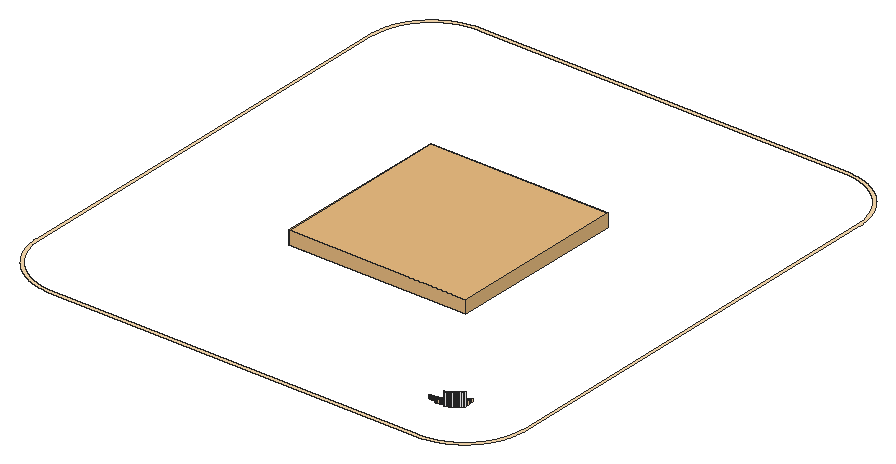
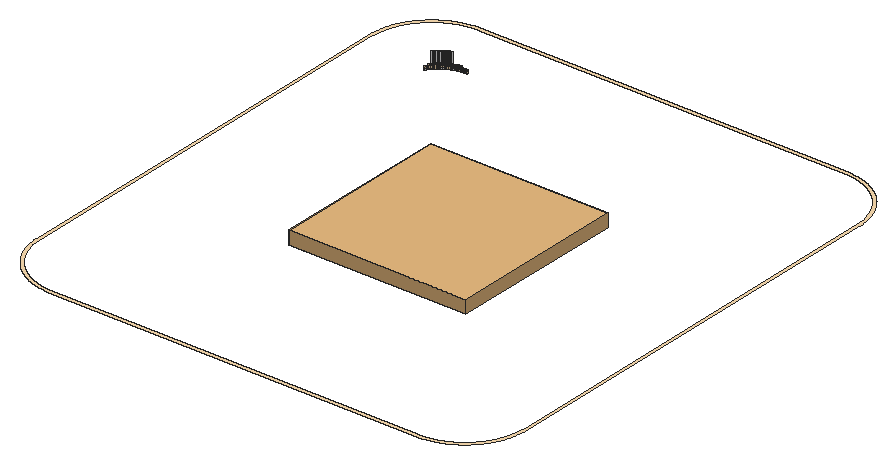
# SketchUp Ruby script. Lengths in inches.
U = 1.inch
M = Sketchup.active_model
def pt(a) = Geom::Point3d.new(a.map { |v| v * U })
def face(e, loops, mat)
  f = e.add_face(loops[0].map { |a| pt(a) })
  loops[1..].each { |l| e.add_face(l.map { |a| pt(a) }).erase! }
  f.material = f.back_material = mat if mat
  f
end
# faces: each face lists its corners as indices into pts; further lists are holes
def faces(e, pts, list, mat = nil) = list.each { |f| face(e, (f[0].is_a?(Array) ? f : [f]).map { |l| l.map { |i| pts[i] } }, mat) }
# xy, xz, yz: faces in a plane at the given z, y or x. An outline is a flat list of corners, or four numbers for a rectangle; further outlines are holes
def ring(l) = l.size == 4 ? [[l[0], l[1]], [l[2], l[1]], [l[2], l[3]], [l[0], l[3]]] : l.each_slice(2).to_a
def flat(e, list, mat, &to3) = list.each { |f| face(e, (f[0].is_a?(Array) ? f : [f]).map { |l| ring(l).map { |u, v| to3.(u, v) } }, mat) }
def xy(e, z, list, mat = nil) = flat(e, list, mat) { |x, y| [x, y, z] }
def xz(e, y, list, mat = nil) = flat(e, list, mat) { |x, z| [x, y, z] }
def yz(e, x, list, mat = nil) = flat(e, list, mat) { |y, z| [x, y, z] }
def lines(e, pts, list) = list.each { |a, b| e.add_line(pt(pts[a]), pt(pts[b])) }
# prism: a flat outline (further loops are holes) pulled along v
def prism(e, loops, v, mat = nil)
  f = face(e, loops, mat); d = Geom::Vector3d.new(v.map { |x| x * U })
  f.pushpull(f.normal.samedirection?(d) ? d.length : -d.length)
end
def box(e, o, s, mat = nil) = prism(e, [[o, [o[0] + s[0], o[1], o[2]], [o[0] + s[0], o[1] + s[1], o[2]], [o[0], o[1] + s[1], o[2]]]], [0, 0, s[2]], mat)
def at(x, y, z, deg = 0) = Geom::Transformation.translation(pt([x, y, z])) * Geom::Transformation.rotation(ORIGIN, Z_AXIS, deg.degrees)
def axes(o, x, y, z) = Geom::Transformation.new([*x, 0, *y, 0, *z, 0, *pt(o).to_a, 1])
def part(name) = M.definitions.add(name)
# library, detail: a bought-in or finely detailed component or shape, given as its bounding box
def library(name, o, s) = part(name).tap { |d| box(d.entities, o, s) }
def detail(e, o, s) = box(e.add_group.entities, o, s)
def put(e, d, t, mat = nil) = e.add_instance(d, t).tap { |i| i.material = mat if mat }
def group(e, t, mat = nil) = e.add_group.tap { |g| g.transformation = t; g.material = mat if mat }.entities
root = M.entities
M.materials.add("False Ceiling Light").color = [254, 223, 179]
M.materials.add("[Quartz Light Grey]").color = [251, 251, 252]
c1 = library("Group\#76",[0,0,0],[64,64,5])
xy(root,116.49,[[[44.53,43.5,177.47,43.5,177.71,43.51,177.94,43.52,178.18,43.53,178.41,43.54,178.65,43.56,178.88,43.58,179.12,43.6,179.35,43.625,179.59,43.65,180.05,43.71,180.29,43.74,180.98,43.86,181.22,43.9,181.45,43.94,182.14,44.09,182.6,44.21,182.82,44.27,183.28,44.39,183.5,44.46,183.73,44.53,183.95,44.6,184.18,44.68,184.4,44.75,184.84,44.91,185.0625,44.99,185.28,45.08,185.72,45.26,185.9375,45.35,186.15,45.45,186.37,45.54,186.79,45.74,187,45.85,187.21,45.95,187.84,46.28,188.05,46.4,188.25,46.51,188.45,46.63,188.66,46.75,188.86,46.88,189.06,47,189.25,47.13,189.65,47.39,189.84,47.52,190.03,47.66,190.23,47.8,190.42,47.9375,190.6,48.08,190.79,48.22,190.98,48.37,191.16,48.51,191.52,48.81,191.7,48.97,191.88,49.12,192.06,49.28,192.23,49.4375,192.4,49.6,192.74,49.92,193.08,50.26,193.4,50.6,193.5625,50.77,193.72,50.94,193.88,51.12,194.03,51.3,194.19,51.48,194.49,51.84,194.63,52.02,194.78,52.21,194.92,52.4,195.0625,52.58,195.2,52.77,195.34,52.97,195.48,53.16,195.61,53.35,195.87,53.75,196,53.94,196.12,54.14,196.25,54.34,196.37,54.55,196.49,54.75,196.6,54.95,196.72,55.16,197.05,55.79,197.15,56,197.26,56.21,197.46,56.63,197.55,56.85,197.65,57.0625,197.74,57.28,197.92,57.72,198.01,57.9375,198.09,58.16,198.25,58.6,198.32,58.82,198.4,59.05,198.47,59.27,198.54,59.5,198.61,59.72,198.73,60.18,198.79,60.4,198.91,60.86,199.06,61.55,199.1,61.78,199.14,62.02,199.26,62.71,199.29,62.95,199.35,63.41,199.375,63.65,199.4,63.88,199.42,64.12,199.44,64.35,199.46,64.59,199.47,64.82,199.48,65.06,199.49,65.29,199.5,65.53,199.5,216.47,199.49,216.71,199.48,216.94,199.47,217.18,199.46,217.41,199.44,217.65,199.42,217.88,199.4,218.12,199.375,218.35,199.35,218.59,199.29,219.05,199.26,219.29,199.14,219.98,199.1,220.22,199.06,220.45,198.91,221.14,198.79,221.6,198.73,221.82,198.61,222.28,198.54,222.5,198.47,222.73,198.4,222.95,198.32,223.18,198.25,223.4,198.09,223.84,198.01,224.0625,197.92,224.28,197.74,224.72,197.65,224.9375,197.55,225.15,197.46,225.37,197.26,225.79,197.15,226,197.05,226.21,196.72,226.84,196.6,227.05,196.49,227.25,196.37,227.45,196.25,227.66,196.12,227.86,196,228.06,195.87,228.25,195.61,228.65,195.48,228.84,195.34,229.03,195.2,229.23,195.0625,229.42,194.92,229.6,194.78,229.79,194.63,229.98,194.49,230.16,194.19,230.52,194.03,230.7,193.88,230.88,193.72,231.06,193.5625,231.23,193.4,231.4,193.08,231.74,192.74,232.08,192.4,232.4,192.23,232.5625,192.06,232.72,191.88,232.88,191.7,233.03,191.52,233.19,191.16,233.49,190.98,233.63,190.79,233.78,190.6,233.92,190.42,234.0625,190.23,234.2,190.03,234.34,189.84,234.48,189.65,234.61,189.25,234.87,189.06,235,188.86,235.12,188.66,235.25,188.45,235.37,188.25,235.49,188.05,235.6,187.84,235.72,187.21,236.05,187,236.15,186.79,236.26,186.37,236.46,186.15,236.55,185.9375,236.65,185.72,236.74,185.28,236.92,185.0625,237.01,184.84,237.09,184.4,237.25,184.18,237.32,183.95,237.4,183.73,237.47,183.5,237.54,183.28,237.61,182.82,237.73,182.6,237.79,182.14,237.91,181.45,238.06,181.22,238.1,180.98,238.14,180.29,238.26,180.05,238.29,179.59,238.35,179.35,238.375,179.12,238.4,178.88,238.42,178.65,238.44,178.41,238.46,178.18,238.47,177.94,238.48,177.71,238.49,177.47,238.5,44.53,238.5,44.29,238.49,44.06,238.48,43.82,238.47,43.59,238.46,43.35,238.44,43.12,238.42,42.88,238.4,42.65,238.375,42.41,238.35,41.95,238.29,41.71,238.26,41.02,238.14,40.78,238.1,40.55,238.06,39.86,237.91,39.4,237.79,39.18,237.73,38.72,237.61,38.5,237.54,38.27,237.47,38.05,237.4,37.82,237.32,37.6,237.25,37.16,237.09,36.9375,237.01,36.72,236.92,36.28,236.74,36.0625,236.65,35.85,236.55,35.63,236.46,35.21,236.26,35,236.15,34.79,236.05,34.16,235.72,33.95,235.6,33.75,235.49,33.55,235.37,33.34,235.25,33.14,235.12,32.94,235,32.75,234.87,32.35,234.61,32.16,234.48,31.97,234.34,31.77,234.2,31.58,234.0625,31.4,233.92,31.21,233.78,31.02,233.63,30.84,233.49,30.48,233.19,30.3,233.03,30.12,232.88,29.94,232.72,29.77,232.5625,29.6,232.4,29.26,232.08,28.92,231.74,28.6,231.4,28.4375,231.23,28.28,231.06,28.12,230.88,27.97,230.7,27.81,230.52,27.51,230.16,27.37,229.98,27.22,229.79,27.08,229.6,26.9375,229.42,26.8,229.23,26.66,229.03,26.52,228.84,26.39,228.65,26.13,228.25,26,228.06,25.88,227.86,25.75,227.66,25.63,227.45,25.51,227.25,25.4,227.05,25.28,226.84,24.95,226.21,24.85,226,24.74,225.79,24.54,225.37,24.45,225.15,24.35,224.9375,24.26,224.72,24.08,224.28,23.99,224.0625,23.91,223.84,23.75,223.4,23.68,223.18,23.6,222.95,23.53,222.73,23.46,222.5,23.39,222.28,23.27,221.82,23.21,221.6,23.09,221.14,22.94,220.45,22.9,220.22,22.86,219.98,22.74,219.29,22.71,219.05,22.65,218.59,22.625,218.35,22.6,218.12,22.58,217.88,22.56,217.65,22.54,217.41,22.53,217.18,22.52,216.94,22.51,216.71,22.5,216.47,22.5,65.53,22.51,65.29,22.52,65.06,22.53,64.82,22.54,64.59,22.56,64.35,22.58,64.12,22.6,63.88,22.625,63.65,22.65,63.41,22.71,62.95,22.74,62.71,22.86,62.02,22.9,61.78,22.94,61.55,23.09,60.86,23.21,60.4,23.27,60.18,23.39,59.72,23.46,59.5,23.53,59.27,23.6,59.05,23.68,58.82,23.75,58.6,23.91,58.16,23.99,57.9375,24.08,57.72,24.26,57.28,24.35,57.0625,24.45,56.85,24.54,56.63,24.74,56.21,24.85,56,24.95,55.79,25.28,55.16,25.4,54.95,25.51,54.75,25.63,54.55,25.75,54.34,25.88,54.14,26,53.94,26.13,53.75,26.39,53.35,26.52,53.16,26.66,52.97,26.8,52.77,26.9375,52.58,27.08,52.4,27.22,52.21,27.37,52.02,27.51,51.84,27.81,51.48,27.97,51.3,28.12,51.12,28.28,50.94,28.4375,50.77,28.6,50.6,28.92,50.26,29.26,49.92,29.6,49.6,29.77,49.4375,29.94,49.28,30.12,49.12,30.3,48.97,30.48,48.81,30.84,48.51,31.02,48.37,31.21,48.22,31.4,48.08,31.58,47.9375,31.77,47.8,31.97,47.66,32.16,47.52,32.35,47.39,32.75,47.13,32.94,47,33.14,46.88,33.34,46.75,33.55,46.63,33.75,46.51,33.95,46.4,34.16,46.28,34.79,45.95,35,45.85,35.21,45.74,35.63,45.54,35.85,45.45,36.0625,45.35,36.28,45.26,36.72,45.08,36.9375,44.99,37.16,44.91,37.6,44.75,37.82,44.68,38.05,44.6,38.27,44.53,38.5,44.46,38.72,44.39,39.18,44.27,39.4,44.21,39.86,44.09,40.55,43.94,40.78,43.9,41.02,43.86,41.71,43.74,41.95,43.71,42.41,43.65,42.65,43.625,42.88,43.6,43.12,43.58,43.35,43.56,43.59,43.54,43.82,43.53,44.06,43.52,44.29,43.51],[44.55,44.5,44.32,44.51,44.1,44.52,43.65,44.54,43.43,44.56,43.2,44.58,42.98,44.6,42.75,44.62,42.53,44.64,42.31,44.67,42.08,44.7,41.64,44.76,41.41,44.8,40.75,44.92,39.87,45.12,39.65,45.18,39.44,45.23,39,45.35,38.79,45.42,38.57,45.48,38.36,45.55,38.14,45.625,37.93,45.7,37.72,45.77,37.09,46.01,36.875,46.09,36.67,46.18,36.46,46.27,36.26,46.36,36.05,46.45,35.85,46.55,35.64,46.64,35.24,46.84,35.04,46.95,34.84,47.05,34.64,47.16,34.45,47.27,34.25,47.38,34.06,47.49,33.86,47.61,33.1,48.09,32.92,48.22,32.73,48.35,32.55,48.47,32.36,48.61,32.18,48.74,31.82,49.01,31.65,49.15,31.47,49.29,31.3,49.43,31.12,49.58,30.95,49.72,30.61,50.02,30.45,50.17,30.28,50.33,30.12,50.48,29.48,51.12,29.33,51.28,29.17,51.45,29.02,51.61,28.72,51.95,28.58,52.12,28.43,52.3,28.29,52.47,28.15,52.65,28.01,52.82,27.74,53.18,27.61,53.36,27.47,53.55,27.35,53.73,27.22,53.92,27.09,54.1,26.61,54.86,26.49,55.06,26.38,55.25,26.27,55.45,26.16,55.64,26.05,55.84,25.95,56.04,25.84,56.24,25.64,56.64,25.55,56.85,25.45,57.05,25.36,57.26,25.27,57.46,25.18,57.67,25.09,57.875,25.01,58.09,24.77,58.72,24.7,58.93,24.625,59.14,24.55,59.36,24.48,59.57,24.42,59.79,24.35,60,24.23,60.44,24.18,60.65,24.12,60.87,23.92,61.75,23.8,62.41,23.76,62.64,23.7,63.08,23.67,63.31,23.64,63.53,23.62,63.75,23.6,63.98,23.58,64.2,23.56,64.43,23.54,64.65,23.52,65.1,23.51,65.32,23.5,65.55,23.5,216.45,23.51,216.68,23.52,216.9,23.54,217.35,23.56,217.57,23.58,217.8,23.6,218.02,23.62,218.25,23.64,218.47,23.67,218.69,23.7,218.92,23.76,219.36,23.8,219.59,23.92,220.25,24.12,221.13,24.18,221.35,24.23,221.56,24.35,222,24.42,222.21,24.48,222.43,24.55,222.64,24.625,222.86,24.7,223.07,24.77,223.28,25.01,223.91,25.09,224.125,25.18,224.33,25.27,224.54,25.36,224.74,25.45,224.95,25.55,225.15,25.64,225.36,25.84,225.76,25.95,225.96,26.05,226.16,26.16,226.36,26.27,226.55,26.38,226.75,26.49,226.94,26.61,227.14,27.09,227.9,27.22,228.08,27.35,228.27,27.47,228.45,27.61,228.64,27.74,228.82,28.01,229.18,28.15,229.35,28.29,229.53,28.43,229.7,28.58,229.88,28.72,230.05,29.02,230.39,29.17,230.55,29.33,230.72,29.48,230.88,30.12,231.52,30.28,231.67,30.45,231.83,30.61,231.98,30.95,232.28,31.12,232.42,31.3,232.57,31.47,232.71,31.65,232.85,31.82,232.99,32.18,233.26,32.36,233.39,32.55,233.53,32.73,233.65,32.92,233.78,33.1,233.91,33.86,234.39,34.06,234.51,34.25,234.62,34.45,234.73,34.64,234.84,34.84,234.95,35.04,235.05,35.24,235.16,35.64,235.36,35.85,235.45,36.05,235.55,36.26,235.64,36.46,235.73,36.67,235.82,36.875,235.91,37.09,235.99,37.72,236.23,37.93,236.3,38.14,236.375,38.36,236.45,38.57,236.52,38.79,236.58,39,236.65,39.44,236.77,39.65,236.82,39.87,236.88,40.75,237.08,41.41,237.2,41.64,237.24,42.08,237.3,42.31,237.33,42.53,237.36,42.75,237.38,42.98,237.4,43.2,237.42,43.43,237.44,43.65,237.46,44.1,237.48,44.32,237.49,44.55,237.5,177.45,237.5,177.68,237.49,177.9,237.48,178.35,237.46,178.57,237.44,178.8,237.42,179.02,237.4,179.25,237.38,179.47,237.36,179.69,237.33,179.92,237.3,180.36,237.24,180.59,237.2,181.25,237.08,182.13,236.88,182.35,236.82,182.56,236.77,183,236.65,183.21,236.58,183.43,236.52,183.64,236.45,183.86,236.375,184.07,236.3,184.28,236.23,184.91,235.99,185.125,235.91,185.33,235.82,185.54,235.73,185.74,235.64,185.95,235.55,186.15,235.45,186.36,235.36,186.76,235.16,186.96,235.05,187.16,234.95,187.36,234.84,187.55,234.73,187.75,234.62,187.94,234.51,188.14,234.39,188.9,233.91,189.08,233.78,189.27,233.65,189.45,233.53,189.64,233.39,189.82,233.26,190.18,232.99,190.35,232.85,190.53,232.71,190.7,232.57,190.88,232.42,191.05,232.28,191.39,231.98,191.55,231.83,191.72,231.67,191.88,231.52,192.52,230.88,192.67,230.72,192.83,230.55,192.98,230.39,193.28,230.05,193.42,229.88,193.57,229.7,193.71,229.53,193.85,229.35,193.99,229.18,194.26,228.82,194.39,228.64,194.53,228.45,194.65,228.27,194.78,228.08,194.91,227.9,195.39,227.14,195.51,226.94,195.62,226.75,195.73,226.55,195.84,226.36,195.95,226.16,196.05,225.96,196.16,225.76,196.36,225.36,196.45,225.15,196.55,224.95,196.64,224.74,196.73,224.54,196.82,224.33,196.91,224.125,196.99,223.91,197.23,223.28,197.3,223.07,197.375,222.86,197.45,222.64,197.52,222.43,197.58,222.21,197.65,222,197.77,221.56,197.82,221.35,197.88,221.13,198.08,220.25,198.2,219.59,198.24,219.36,198.3,218.92,198.33,218.69,198.36,218.47,198.38,218.25,198.4,218.02,198.42,217.8,198.44,217.57,198.46,217.35,198.48,216.9,198.49,216.68,198.5,216.45,198.5,65.55,198.49,65.32,198.48,65.1,198.46,64.65,198.44,64.43,198.42,64.2,198.4,63.98,198.38,63.75,198.36,63.53,198.33,63.31,198.3,63.08,198.24,62.64,198.2,62.41,198.08,61.75,197.88,60.87,197.82,60.65,197.77,60.44,197.65,60,197.58,59.79,197.52,59.57,197.45,59.36,197.375,59.14,197.3,58.93,197.23,58.72,196.99,58.09,196.91,57.875,196.82,57.67,196.73,57.46,196.64,57.26,196.55,57.05,196.45,56.85,196.36,56.64,196.16,56.24,196.05,56.04,195.95,55.84,195.84,55.64,195.73,55.45,195.62,55.25,195.51,55.06,195.39,54.86,194.91,54.1,194.78,53.92,194.65,53.73,194.53,53.55,194.39,53.36,194.26,53.18,193.99,52.82,193.85,52.65,193.71,52.47,193.57,52.3,193.42,52.12,193.28,51.95,192.98,51.61,192.83,51.45,192.67,51.28,192.52,51.12,191.88,50.48,191.72,50.33,191.55,50.17,191.39,50.02,191.05,49.72,190.88,49.58,190.7,49.43,190.53,49.29,190.35,49.15,190.18,49.01,189.82,48.74,189.64,48.61,189.45,48.47,189.27,48.35,189.08,48.22,188.9,48.09,188.14,47.61,187.94,47.49,187.75,47.38,187.55,47.27,187.36,47.16,187.16,47.05,186.96,46.95,186.76,46.84,186.36,46.64,186.15,46.55,185.95,46.45,185.74,46.36,185.54,46.27,185.33,46.18,185.125,46.09,184.91,46.01,184.28,45.77,184.07,45.7,183.86,45.625,183.64,45.55,183.43,45.48,183.21,45.42,183,45.35,182.56,45.23,182.35,45.18,182.13,45.12,181.25,44.92,180.59,44.8,180.36,44.76,179.92,44.7,179.69,44.67,179.47,44.64,179.25,44.62,179.02,44.6,178.8,44.58,178.57,44.56,178.35,44.54,177.9,44.52,177.68,44.51,177.45,44.5]]],"False Ceiling Light")
xz(root,64.5,[[165,115.32,165.18,116.49],[165.18,115.32,165.35,116.49]],"False Ceiling Light")
xz(root,64.5,[[165,115.32,165.18,115.91],[165.18,115.32,165.35,115.91]],"[Quartz Light Grey]")
p = [[167.83,63.78,115.32],[168.01,63.82,115.32],[168.01,63.82,116.49],[167.83,63.78,116.49],[168.2,63.86,115.32],[168.2,63.86,116.49],
  [171.3,63.84,115.32],[171.12,63.76,115.32],[171.12,63.76,120],[171.3,63.84,120],[171.49,63.92,115.32],[171.49,63.92,120],
  [168.38,63.9,115.32],[168.38,63.9,116.49],[168.57,63.95,115.32],[168.57,63.95,116.49],[168.75,63.99,115.32],[168.75,63.99,116.49],
  [171.67,64.01,115.32],[171.67,64.01,120],[168.9375,64.04,115.32],[168.9375,64.04,116.49],[169.12,64.1,115.32],[169.12,64.1,116.49],
  [171.86,64.1,115.32],[171.86,64.1,120],[169.3,64.15,115.32],[169.3,64.15,116.49],[172.04,64.1875,115.32],[172.04,64.1875,120],
  [169.48,64.21,115.32],[169.48,64.21,116.49],[169.66,64.27,115.32],[169.66,64.27,116.49],[172.22,64.28,115.32],[172.22,64.28,120],
  [169.84,64.33,115.32],[169.84,64.33,116.49],[170.02,64.4,115.32],[170.02,64.4,116.49],[172.4,64.38,115.32],[172.4,64.38,120],
  [170.2,64.46,115.32],[170.2,64.46,116.49],[172.57,64.48,115.32],[172.57,64.48,120],[165.53,64.51,115.32],[165.35,64.5,115.32],
  [165.35,64.5,116.49],[165.53,64.51,116.49],[165.35,64.5,115.32],[165.53,64.51,115.32],[165.53,64.51,115.91],[165.35,64.5,115.91],
  [165.71,64.52,115.32],[165.71,64.52,116.49],[165.71,64.52,115.32],[165.71,64.52,115.91],[165.88,64.53,115.32],[165.88,64.53,116.49],
  [165.88,64.53,115.32],[165.88,64.53,115.91],[166.06,64.54,115.32],[166.06,64.54,116.49],[166.06,64.54,115.32],[166.06,64.54,115.91],
  [166.24,64.56,115.32],[166.24,64.56,116.49],[166.24,64.56,115.32],[166.24,64.56,115.91],[170.375,64.53,115.32],[170.375,64.53,116.49],
  [170.55,64.6,115.32],[170.55,64.6,116.49],[172.75,64.58,115.32],[172.75,64.58,120],[166.41,64.57,115.32],[166.41,64.57,116.49],
  [166.41,64.57,115.32],[166.41,64.57,115.91],[166.59,64.59,115.32],[166.59,64.59,116.49],[166.59,64.59,115.32],[166.59,64.59,115.91],
  [166.76,64.62,115.32],[166.76,64.62,116.49],[166.76,64.62,115.32],[166.76,64.62,115.91],[166.9375,64.64,115.32],[166.9375,64.64,116.49],
  [166.9375,64.64,115.32],[166.9375,64.64,115.91],[167.11,64.67,115.32],[167.11,64.67,116.49],[167.11,64.67,115.32],[167.11,64.67,115.91],
  [170.72,64.68,115.32],[170.72,64.68,116.49],[172.93,64.68,115.32],[172.93,64.68,120],[167.29,64.69,115.32],[167.29,64.69,116.49],
  [167.29,64.69,115.32],[167.29,64.69,115.91],[167.46,64.73,115.32],[167.46,64.73,116.49],[167.46,64.73,115.32],[167.46,64.73,115.91],
  [167.63,64.76,115.32],[167.63,64.76,116.49],[167.63,64.76,115.32],[167.63,64.76,115.91],[170.9,64.75,115.32],[170.9,64.75,116.49],
  [173.1,64.78,115.32],[173.1,64.78,120],[167.81,64.79,115.32],[167.81,64.79,116.49],[167.81,64.79,115.32],[167.81,64.79,115.91],
  [167.98,64.83,115.32],[167.98,64.83,116.49],[167.98,64.83,115.32],[167.98,64.83,115.91],[168.15,64.87,115.32],[168.15,64.87,116.49],
  [168.15,64.87,115.32],[168.15,64.87,115.91],[171.07,64.83,115.32],[171.07,64.83,116.49],[171.24,64.91,115.32],[171.24,64.91,116.49],
  [173.27,64.89,115.32],[173.27,64.89,120],[168.32,64.92,115.32],[168.32,64.92,116.49],[168.32,64.92,115.32],[168.32,64.92,115.91],
  [168.49,64.96,115.32],[168.49,64.96,116.49],[168.49,64.96,115.32],[168.49,64.96,115.91],[171.41,65,115.32],[171.41,65,116.49],
  [173.44,65,115.32],[173.44,65,120],[168.66,65.01,115.32],[168.66,65.01,116.49],[168.66,65.01,115.32],[168.66,65.01,115.91],
  [168.83,65.06,115.32],[168.83,65.06,116.49],[168.83,65.06,115.32],[168.83,65.06,115.91],[171.58,65.08,115.32],[171.58,65.08,116.49],
  [173.61,65.11,115.32],[173.61,65.11,120],[169,65.11,115.32],[169,65.11,116.49],[169,65.11,115.32],[169,65.11,115.91],
  [169.17,65.16,115.32],[169.17,65.16,116.49],[169.17,65.16,115.32],[169.17,65.16,115.91],[171.75,65.17,115.32],[171.75,65.17,116.49],
  [173.78,65.23,115.32],[173.78,65.23,120],[169.34,65.22,115.32],[169.34,65.22,116.49],[169.34,65.22,115.32],[169.34,65.22,115.91],
  [169.51,65.27,115.32],[169.51,65.27,116.49],[169.51,65.27,115.32],[169.51,65.27,115.91],[171.92,65.26,115.32],[171.92,65.26,116.49],
  [173.95,65.34,115.32],[173.95,65.34,120],[169.67,65.33,115.32],[169.67,65.33,116.49],[169.67,65.33,115.32],[169.67,65.33,115.91],
  [169.84,65.4,115.32],[169.84,65.4,116.49],[169.84,65.4,115.32],[169.84,65.4,115.91],[172.09,65.35,115.32],[172.09,65.35,116.49],
  [172.25,65.44,115.32],[172.25,65.44,116.49],[174.11,65.46,115.32],[174.11,65.46,120],[170,65.46,115.32],[170,65.46,116.49],
  [170,65.46,115.32],[170,65.46,115.91],[172.41,65.54,115.32],[172.41,65.54,116.49],[170.17,65.53,115.32],[170.17,65.53,116.49],
  [170.17,65.53,115.32],[170.17,65.53,115.91],[170.33,65.6,115.32],[170.33,65.6,116.49],[170.33,65.6,115.32],[170.33,65.6,115.91],
  [172.58,65.64,115.32],[172.58,65.64,116.49],[174.27,65.58,115.32],[174.27,65.58,120],[170.49,65.67,115.32],[170.49,65.67,116.49],
  [170.49,65.67,115.32],[170.49,65.67,115.91],[172.74,65.74,115.32],[172.74,65.74,116.49],[174.4375,65.7,115.32],[174.4375,65.7,120],
  [170.65,65.74,115.32],[170.65,65.74,116.49],[170.65,65.74,115.32],[170.65,65.74,115.91],[170.8125,65.82,115.32],[170.8125,65.82,116.49],
  [170.8125,65.82,115.32],[170.8125,65.82,115.91],[172.9,65.84,115.32],[172.9,65.84,116.49],[174.6,65.83,115.32],[174.6,65.83,120],
  [170.97,65.89,115.32],[170.97,65.89,116.49],[170.97,65.89,115.32],[170.97,65.89,115.91],[173.06,65.94,115.32],[173.06,65.94,116.49],
  [174.75,65.95,115.32],[174.75,65.95,120],[171.13,65.97,115.32],[171.13,65.97,116.49],[171.13,65.97,115.32],[171.13,65.97,115.91],
  [173.21,66.05,115.32],[173.21,66.05,116.49],[171.29,66.05,115.32],[171.29,66.05,116.49],[171.29,66.05,115.32],[171.29,66.05,115.91],
  [174.91,66.08,115.32],[174.91,66.08,120],[171.44,66.14,115.32],[171.44,66.14,116.49],[171.44,66.14,115.32],[171.44,66.14,115.91],
  [171.6,66.22,115.32],[171.6,66.22,116.49],[171.6,66.22,115.32],[171.6,66.22,115.91],[173.37,66.16,115.32],[173.37,66.16,116.49],
  [175.07,66.21,115.32],[175.07,66.21,120],[171.75,66.31,115.32],[171.75,66.31,116.49],[171.75,66.31,115.32],[171.75,66.31,115.91],
  [173.52,66.27,115.32],[173.52,66.27,116.49],[175.22,66.35,115.32],[175.22,66.35,120],[171.9,66.4,115.32],[171.9,66.4,116.49],
  [171.9,66.4,115.32],[171.9,66.4,115.91],[173.68,66.38,115.32],[173.68,66.38,116.49],[175.37,66.48,115.32],[175.37,66.48,120],
  [172.05,66.49,115.32],[172.05,66.49,116.49],[172.05,66.49,115.32],[172.05,66.49,115.91],[173.83,66.5,115.32],[173.83,66.5,116.49],
  [172.2,66.58,115.32],[172.2,66.58,116.49],[172.2,66.58,115.32],[172.2,66.58,115.91],[173.98,66.61,115.32],[173.98,66.61,116.49],
  [175.52,66.62,115.32],[175.52,66.62,120],[172.35,66.68,115.32],[172.35,66.68,116.49],[172.35,66.68,115.32],[172.35,66.68,115.91],
  [174.125,66.73,115.32],[174.125,66.73,116.49],[175.67,66.76,115.32],[175.67,66.76,120],[172.5,66.78,115.32],[172.5,66.78,116.49],
  [172.5,66.78,115.32],[172.5,66.78,115.91],[174.27,66.85,115.32],[174.27,66.85,116.49],[172.65,66.875,115.32],[172.65,66.875,116.49],
  [172.65,66.875,115.32],[172.65,66.875,115.91],[175.82,66.9,115.32],[175.82,66.9,120],[172.79,66.98,115.32],[172.79,66.98,116.49],
  [172.79,66.98,115.32],[172.79,66.98,115.91],[174.42,66.97,115.32],[174.42,66.97,116.49],[175.96,67.04,115.32],[175.96,67.04,120],
  [172.94,67.08,115.32],[172.94,67.08,116.49],[172.94,67.08,115.32],[172.94,67.08,115.91],[174.5625,67.1,115.32],[174.5625,67.1,116.49],
  [176.1,67.18,115.32],[176.1,67.18,120],[173.08,67.18,115.32],[173.08,67.18,116.49],[173.08,67.18,115.32],[173.08,67.18,115.91],
  [174.7,67.22,115.32],[174.7,67.22,116.49],[173.22,67.29,115.32],[173.22,67.29,116.49],[173.22,67.29,115.32],[173.22,67.29,115.91],
  [174.84,67.35,115.32],[174.84,67.35,116.49],[176.24,67.33,115.32],[176.24,67.33,120],[173.36,67.4,115.32],[173.36,67.4,116.49],
  [173.36,67.4,115.32],[173.36,67.4,115.91],[173.5,67.51,115.32],[173.5,67.51,116.49],[173.5,67.51,115.32],[173.5,67.51,115.91],
  [174.98,67.48,115.32],[174.98,67.48,116.49],[173.63,67.62,115.32],[173.63,67.62,116.49],[173.63,67.62,115.32],[173.63,67.62,115.91],
  [175.12,67.61,115.32],[175.12,67.61,116.49],[173.77,67.73,115.32],[173.77,67.73,116.49],[173.77,67.73,115.32],[173.77,67.73,115.91],
  [175.25,67.75,115.32],[175.25,67.75,116.49],[173.9,67.85,115.32],[173.9,67.85,116.49],[173.9,67.85,115.32],[173.9,67.85,115.91],
  [175.39,67.88,115.32],[175.39,67.88,116.49],[174.03,67.97,115.32],[174.03,67.97,116.49],[174.03,67.97,115.32],[174.03,67.97,115.91],
  [175.52,68.02,115.32],[175.52,68.02,116.49],[174.16,68.09,115.32],[174.16,68.09,116.49],[174.16,68.09,115.32],[174.16,68.09,115.91],
  [175.65,68.16,115.32],[175.65,68.16,116.49],[174.29,68.21,115.32],[174.29,68.21,116.49],[174.29,68.21,115.32],[174.29,68.21,115.91],
  [174.42,68.33,115.32],[174.42,68.33,116.49],[174.42,68.33,115.32],[174.42,68.33,115.91],[175.78,68.3,115.32],[175.78,68.3,116.49],
  [174.55,68.45,115.32],[174.55,68.45,116.49],[174.55,68.45,115.32],[174.55,68.45,115.91],[175.9,68.4375,115.32],[175.9,68.4375,116.49],
  [176.03,68.58,115.32],[176.03,68.58,116.49],[174.67,68.58,115.32],[174.67,68.58,116.49],[174.67,68.58,115.32],[174.67,68.58,115.91],
  [174.79,68.71,115.32],[174.79,68.71,116.49],[174.79,68.71,115.32],[174.79,68.71,115.91],[176.15,68.73,115.32],[176.15,68.73,116.49],
  [174.91,68.84,115.32],[174.91,68.84,116.49],[174.91,68.84,115.32],[174.91,68.84,115.91],[175.03,68.97,115.32],[175.03,68.97,116.49],
  [175.03,68.97,115.32],[175.03,68.97,115.91],[175.15,69.1,115.32],[175.15,69.1,116.49],[175.15,69.1,115.32],[175.15,69.1,115.91],
  [175.27,69.23,115.32],[175.27,69.23,116.49],[175.27,69.23,115.32],[175.27,69.23,115.91],[175.38,69.37,115.32],[175.38,69.37,116.49],
  [175.38,69.37,115.32],[175.38,69.37,115.91],[175.49,69.5,115.32],[175.49,69.5,116.49],[175.49,69.5,115.32],[175.49,69.5,115.91],
  [175.6,69.64,115.32],[175.6,69.64,116.49],[175.6,69.64,115.32],[175.6,69.64,115.91],[175.71,69.78,115.32],[175.71,69.78,116.49],
  [175.71,69.78,115.32],[175.71,69.78,115.91],[175.82,69.92,115.32],[175.82,69.92,116.49],[175.82,69.92,115.32],[175.82,69.92,115.91],
  [175.92,70.06,115.32],[175.92,70.06,116.49],[175.92,70.06,115.32],[175.92,70.06,115.91],[176.02,70.21,115.32],[176.02,70.21,116.49],
  [176.02,70.21,115.32],[176.02,70.21,115.91],[176.125,70.35,115.32],[176.125,70.35,116.49],[176.125,70.35,115.32],[176.125,70.35,115.91],
  [176.22,70.5,115.32],[176.22,70.5,116.49],[176.22,70.5,115.32],[176.22,70.5,115.91]]
faces(root,p,[[0,1,2,3],[1,4,5,2],[4,12,13,5],[12,14,15,13],[14,16,17,15],[16,20,21,17],[20,22,23,21],[22,26,27,23],
  [26,30,31,27],[30,32,33,31],[32,36,37,33],[36,38,39,37],[38,42,43,39],[46,47,48,49],[54,46,49,55],[58,54,55,59],
  [62,58,59,63],[66,62,63,67],[42,70,71,43],[70,72,73,71],[76,66,67,77],[80,76,77,81],[84,80,81,85],[88,84,85,89],
  [92,88,89,93],[72,96,97,73],[100,92,93,101],[104,100,101,105],[108,104,105,109],[96,112,113,97],[116,108,109,117],[120,116,117,121],
  [124,120,121,125],[112,128,129,113],[128,130,131,129],[134,124,125,135],[138,134,135,139],[130,142,143,131],[146,138,139,147],[150,146,147,151],
  [142,154,155,143],[158,150,151,159],[162,158,159,163],[154,166,167,155],[170,162,163,171],[174,170,171,175],[166,178,179,167],[182,174,175,183],
  [186,182,183,187],[178,190,191,179],[190,192,193,191],[196,186,187,197],[192,200,201,193],[202,196,197,203],[206,202,203,207],[200,210,211,201],
  [214,206,207,215],[210,218,219,211],[222,214,215,223],[226,222,223,227],[218,230,231,219],[234,226,227,235],[230,238,239,231],[242,234,235,243],
  [238,246,247,239],[248,242,243,249],[254,248,249,255],[258,254,255,259],[246,262,263,247],[266,258,259,267],[262,270,271,263],[274,266,267,275],
  [270,278,279,271],[282,274,275,283],[278,286,287,279],[288,282,283,289],[286,292,293,287],[296,288,289,297],[292,300,301,293],[304,296,297,305],
  [300,308,309,301],[310,304,305,311],[316,310,311,317],[308,320,321,309],[324,316,317,325],[320,328,329,321],[332,324,325,333],[328,336,337,329],
  [338,332,333,339],[336,342,343,337],[346,338,339,347],[350,346,347,351],[342,354,355,343],[356,350,351,357],[354,360,361,355],[362,356,357,363],
  [360,366,367,361],[368,362,363,369],[366,372,373,367],[374,368,369,375],[372,378,379,373],[380,374,375,381],[378,384,385,379],[386,380,381,387],
  [390,386,387,391],[384,394,395,385],[396,390,391,397],[394,400,401,395],[400,402,403,401],[404,396,397,405],[408,404,405,409],[402,412,413,403],
  [414,408,409,415],[418,414,415,419],[422,418,419,423],[426,422,423,427],[430,426,427,431],[434,430,431,435],[438,434,435,439],[442,438,439,443],
  [446,442,443,447],[450,446,447,451],[454,450,451,455],[458,454,455,459],[462,458,459,463]],"False Ceiling Light")
faces(root,p,[[6,7,8,9],[10,6,9,11],[18,10,11,19],[24,18,19,25],[28,24,25,29],[34,28,29,35],[40,34,35,41],[44,40,41,45],
  [50,51,52,53],[51,56,57,52],[56,60,61,57],[60,64,65,61],[64,68,69,65],[74,44,45,75],[68,78,79,69],[78,82,83,79],
  [82,86,87,83],[86,90,91,87],[90,94,95,91],[98,74,75,99],[94,102,103,95],[102,106,107,103],[106,110,111,107],[114,98,99,115],
  [110,118,119,111],[118,122,123,119],[122,126,127,123],[132,114,115,133],[126,136,137,127],[136,140,141,137],[144,132,133,145],[140,148,149,141],
  [148,152,153,149],[156,144,145,157],[152,160,161,153],[160,164,165,161],[168,156,157,169],[164,172,173,165],[172,176,177,173],[180,168,169,181],
  [176,184,185,177],[184,188,189,185],[194,180,181,195],[188,198,199,189],[198,204,205,199],[204,208,209,205],[212,194,195,213],[208,216,217,209],
  [220,212,213,221],[216,224,225,217],[224,228,229,225],[232,220,221,233],[228,236,237,229],[240,232,233,241],[236,244,245,237],[244,250,251,245],
  [252,240,241,253],[250,256,257,251],[256,260,261,257],[264,252,253,265],[260,268,269,261],[272,264,265,273],[268,276,277,269],[280,272,273,281],
  [276,284,285,277],[284,290,291,285],[294,280,281,295],[290,298,299,291],[302,294,295,303],[298,306,307,299],[306,312,313,307],[314,302,303,315],
  [312,318,319,313],[322,314,315,323],[318,326,327,319],[330,322,323,331],[326,334,335,327],[334,340,341,335],[344,330,331,345],[340,348,349,341],
  [348,352,353,349],[352,358,359,353],[358,364,365,359],[364,370,371,365],[370,376,377,371],[376,382,383,377],[382,388,389,383],[388,392,393,389],
  [392,398,399,393],[398,406,407,399],[406,410,411,407],[410,416,417,411],[416,420,421,417],[420,424,425,421],[424,428,429,425],[428,432,433,429],
  [432,436,437,433],[436,440,441,437],[440,444,445,441],[444,448,449,445],[448,452,453,449],[452,456,457,453],[456,460,461,457],[460,464,465,461]],"[Quartz Light Grey]")
put(root,c1,axes([143,109,115.28],[0,1,0],[-1,0,0],[0,0,0.945]))
